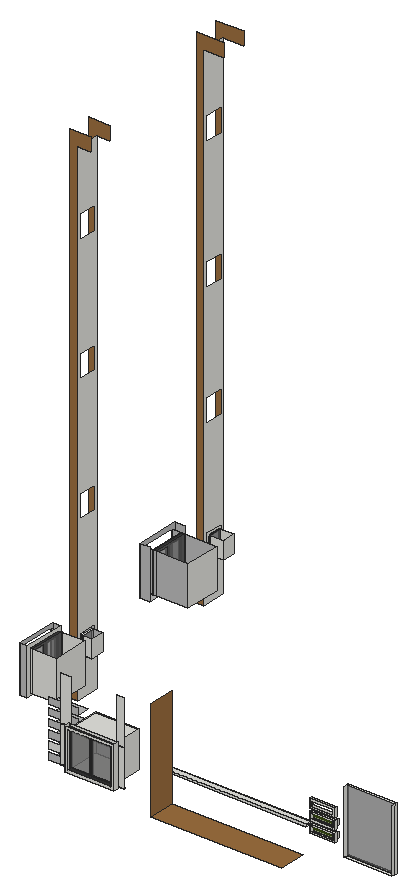
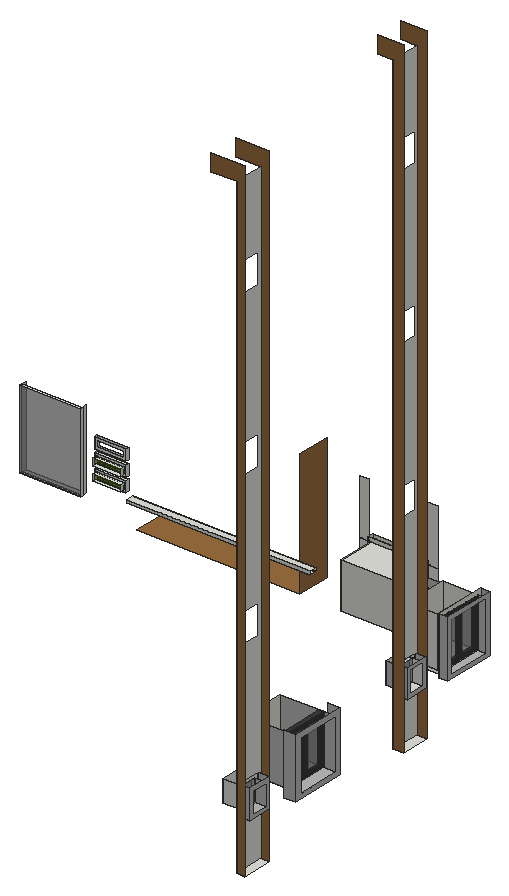
# SketchUp Ruby script. Lengths in inches.
U = 1.inch
M = Sketchup.active_model
def pt(a) = Geom::Point3d.new(a.map { |v| v * U })
def face(e, loops, mat)
  f = e.add_face(loops[0].map { |a| pt(a) })
  loops[1..].each { |l| e.add_face(l.map { |a| pt(a) }).erase! }
  f.material = f.back_material = mat if mat
  f
end
# faces: each face lists its corners as indices into pts; further lists are holes
def faces(e, pts, list, mat = nil) = list.each { |f| face(e, (f[0].is_a?(Array) ? f : [f]).map { |l| l.map { |i| pts[i] } }, mat) }
# xy, xz, yz: faces in a plane at the given z, y or x. An outline is a flat list of corners, or four numbers for a rectangle; further outlines are holes
def ring(l) = l.size == 4 ? [[l[0], l[1]], [l[2], l[1]], [l[2], l[3]], [l[0], l[3]]] : l.each_slice(2).to_a
def flat(e, list, mat, &to3) = list.each { |f| face(e, (f[0].is_a?(Array) ? f : [f]).map { |l| ring(l).map { |u, v| to3.(u, v) } }, mat) }
def xy(e, z, list, mat = nil) = flat(e, list, mat) { |x, y| [x, y, z] }
def xz(e, y, list, mat = nil) = flat(e, list, mat) { |x, z| [x, y, z] }
def yz(e, x, list, mat = nil) = flat(e, list, mat) { |y, z| [x, y, z] }
def lines(e, pts, list) = list.each { |a, b| e.add_line(pt(pts[a]), pt(pts[b])) }
# prism: a flat outline (further loops are holes) pulled along v
def prism(e, loops, v, mat = nil)
  f = face(e, loops, mat); d = Geom::Vector3d.new(v.map { |x| x * U })
  f.pushpull(f.normal.samedirection?(d) ? d.length : -d.length)
end
def box(e, o, s, mat = nil) = prism(e, [[o, [o[0] + s[0], o[1], o[2]], [o[0] + s[0], o[1] + s[1], o[2]], [o[0], o[1] + s[1], o[2]]]], [0, 0, s[2]], mat)
def at(x, y, z, deg = 0) = Geom::Transformation.translation(pt([x, y, z])) * Geom::Transformation.rotation(ORIGIN, Z_AXIS, deg.degrees)
def axes(o, x, y, z) = Geom::Transformation.new([*x, 0, *y, 0, *z, 0, *pt(o).to_a, 1])
def part(name) = M.definitions.add(name)
# library, detail: a bought-in or finely detailed component or shape, given as its bounding box
def library(name, o, s) = part(name).tap { |d| box(d.entities, o, s) }
def detail(e, o, s) = box(e.add_group.entities, o, s)
def put(e, d, t, mat = nil) = e.add_instance(d, t).tap { |i| i.material = mat if mat }
def group(e, t, mat = nil) = e.add_group.tap { |g| g.transformation = t; g.material = mat if mat }.entities
root = M.entities
M.materials.add("Generic").color = [155, 110, 63]
M.materials.add("Generic\#2").color = [186, 186, 186]
M.materials.add("[Color M07]").color = [58, 58, 58]
M.materials.add("[Translucent Glass Dark Green]").color = [62, 91, 5]
M.materials["[Translucent Glass Dark Green]"].alpha = 0.5
M.materials.add("[Translucent Glass Gray]").color = [127, 127, 127]
M.materials["[Translucent Glass Gray]"].alpha = 0.58
M.materials.add("[Translucent Glass Gray]1").color = [127, 127, 127]
M.materials["[Translucent Glass Gray]1"].alpha = 0.5
c1 = part("Group\#1")
xy(c1.entities,0,[[0,0,46.77,20.375]])
xz(c1.entities,0,[[0,0,46.77,11.0625]])
c2 = part("Group\#3")
xy(c2.entities,0,[[0,0,70.4375,6]],"[Color M07]")
xy(c2.entities,2.83,[[2.83,0,33.8,3],[36.63,0,67.61,3]],"[Color M07]")
xy(c2.entities,56.73,[[2.83,0,33.8,3],[36.63,0,67.61,3]],"[Color M07]")
xy(c2.entities,59.5625,[[0,0,70.4375,6]],"[Color M07]")
xz(c2.entities,0,[[[0,0,70.4375,59.5625],[2.83,2.83,33.8,56.73],[36.63,2.83,67.61,56.73]]],"[Color M07]")
xz(c2.entities,3,[[2.83,2.83,33.8,56.73],[36.63,2.83,67.61,56.73]],"[Translucent Glass Gray]")
xz(c2.entities,6,[[0,0,70.4375,59.5625]],"[Translucent Glass Gray]")
yz(c2.entities,0,[[0,0,6,59.5625]],"[Color M07]")
yz(c2.entities,2.83,[[0,2.83,3,56.73]],"[Color M07]")
yz(c2.entities,33.8,[[0,2.83,3,56.73]],"[Color M07]")
yz(c2.entities,36.63,[[0,2.83,3,56.73]],"[Color M07]")
yz(c2.entities,67.61,[[0,2.83,3,56.73]],"[Color M07]")
yz(c2.entities,70.4375,[[0,0,6,59.5625]],"[Color M07]")
c3 = part("Group\#7")
xy(c3.entities,0,[[0,0,36.1875,3]])
xy(c3.entities,8.75,[[0,0,36.1875,3]])
xz(c3.entities,0,[[0,0,36.1875,8.75]],"[Translucent Glass Dark Green]")
xz(c3.entities,3,[[0,0,36.1875,8.75]],"[Translucent Glass Dark Green]")
yz(c3.entities,0,[[0,0,3,8.75]])
yz(c3.entities,36.1875,[[0,0,3,8.75]])
c4 = part("Group\#4")
xy(c4.entities,0,[[0,0,6,57.4375]],"[Color M07]")
xy(c4.entities,5.48,[[0,5.48,3,25.98],[0,31.46,3,51.96]],"[Color M07]")
xy(c4.entities,59.46,[[0,5.48,3,25.98],[0,31.46,3,51.96]],"[Color M07]")
xy(c4.entities,64.9375,[[0,0,6,57.4375]],"[Color M07]")
xz(c4.entities,0,[[0,0,6,64.9375]],"[Color M07]")
xz(c4.entities,5.48,[[0,5.48,3,59.46]],"[Color M07]")
xz(c4.entities,25.98,[[0,5.48,3,59.46]],"[Color M07]")
xz(c4.entities,31.46,[[0,5.48,3,59.46]],"[Color M07]")
xz(c4.entities,51.96,[[0,5.48,3,59.46]],"[Color M07]")
xz(c4.entities,57.4375,[[0,0,6,64.9375]],"[Color M07]")
yz(c4.entities,0,[[[0,0,57.4375,64.9375],[31.46,5.48,51.96,59.46],[5.48,5.48,25.98,59.46]]],"[Color M07]")
yz(c4.entities,3,[[5.48,5.48,25.98,59.46],[31.46,5.48,51.96,59.46]],"[Translucent Glass Gray]1")
yz(c4.entities,6,[[0,0,57.4375,64.9375]],"[Translucent Glass Gray]1")
c5 = part("Group\#5")
xy(c5.entities,0,[[0,0,3,21.5625]])
xy(c5.entities,28.3125,[[0,0,3,21.5625]])
xz(c5.entities,0,[[0,0,3,28.3125]])
xz(c5.entities,21.5625,[[0,0,3,28.3125]])
yz(c5.entities,0,[[0,0,21.5625,28.3125]],"[Translucent Glass Gray]1")
yz(c5.entities,3,[[0,0,21.5625,28.3125]],"[Translucent Glass Gray]1")
xy(root,216.21,[[4.375,563.94,15.3125,603.53]])
xy(root,219.07,[[35,268.32,48.5,306.87]])
xy(root,226.375,[[315.5625,81.125,528.75,124.5]],"Generic")
xy(root,236.625,[[170.35,89.25,249.19,97.25],[172.53,97.25,173.03,98],[247.78,97.25,248.28,98.375]])
xy(root,239.9375,[[157.47,97.25,170.35,98],[249.19,97.25,259.3125,98.375]])
xy(root,240.4375,[[157.47,97.25,170.35,98],[249.19,97.25,259.3125,98.375]])
xy(root,240.83,[[174.55,89.25,244.99,97.25],[174.55,97.25,244.99,145.8125]])
xy(root,246.29,[[594.67,124.5,673.48,130.75]])
xy(root,264.83,[[[290.4375,130.75,528.75,140.05],[520.27,135.31,520.48,135.34,520.67,135.42,520.84,135.55,520.97,135.72,521.05,135.91,521.08,136.12,521.05,136.33,520.97,136.53,520.84,136.7,520.67,136.83,520.48,136.91,520.27,136.93,520.06,136.91,519.86,136.83,519.69,136.7,519.5625,136.53,519.48,136.33,519.45,136.12,519.48,135.91,519.5625,135.72,519.69,135.55,519.86,135.42,520.06,135.34],[514.2,135.31,514.41,135.34,514.61,135.42,514.78,135.55,514.91,135.72,514.99,135.91,515.02,136.12,514.99,136.33,514.91,136.53,514.78,136.7,514.61,136.83,514.41,136.91,514.2,136.93,513.99,136.91,513.8,136.83,513.63,136.7,513.5,136.53,513.42,136.33,513.39,136.12,513.42,135.91,513.5,135.72,513.63,135.55,513.8,135.42,513.99,135.34],[508.14,135.31,508.35,135.34,508.55,135.42,508.72,135.55,508.85,135.72,508.93,135.91,508.95,136.12,508.93,136.33,508.85,136.53,508.72,136.7,508.55,136.83,508.35,136.91,508.14,136.93,507.93,136.91,507.74,136.83,507.57,136.7,507.4375,136.53,507.36,136.33,507.33,136.12,507.36,135.91,507.4375,135.72,507.57,135.55,507.74,135.42,507.93,135.34],[502.27,135.31,502.48,135.34,502.67,135.42,502.84,135.55,502.97,135.72,503.05,135.91,503.08,136.12,503.05,136.33,502.97,136.53,502.84,136.7,502.67,136.83,502.48,136.91,502.27,136.93,502.06,136.91,501.86,136.83,501.69,136.7,501.5625,136.53,501.48,136.33,501.45,136.12,501.48,135.91,501.5625,135.72,501.69,135.55,501.86,135.42,502.06,135.34],[496.27,135.31,496.48,135.34,496.67,135.42,496.84,135.55,496.97,135.72,497.05,135.91,497.08,136.12,497.05,136.33,496.97,136.53,496.84,136.7,496.67,136.83,496.48,136.91,496.27,136.93,496.06,136.91,495.86,136.83,495.69,136.7,495.5625,136.53,495.48,136.33,495.45,136.12,495.48,135.91,495.5625,135.72,495.69,135.55,495.86,135.42,496.06,135.34],[490.27,135.31,490.48,135.34,490.67,135.42,490.84,135.55,490.97,135.72,491.05,135.91,491.08,136.12,491.05,136.33,490.97,136.53,490.84,136.7,490.67,136.83,490.48,136.91,490.27,136.93,490.06,136.91,489.86,136.83,489.69,136.7,489.5625,136.53,489.48,136.33,489.45,136.12,489.48,135.91,489.5625,135.72,489.69,135.55,489.86,135.42,490.06,135.34],[484.2,135.31,484.41,135.34,484.61,135.42,484.78,135.55,484.91,135.72,484.99,135.91,485.02,136.12,484.99,136.33,484.91,136.53,484.78,136.7,484.61,136.83,484.41,136.91,484.2,136.93,483.99,136.91,483.8,136.83,483.63,136.7,483.5,136.53,483.42,136.33,483.39,136.12,483.42,135.91,483.5,135.72,483.63,135.55,483.8,135.42,483.99,135.34],[478.27,135.31,478.48,135.34,478.67,135.42,478.84,135.55,478.97,135.72,479.05,135.91,479.08,136.12,479.05,136.33,478.97,136.53,478.84,136.7,478.67,136.83,478.48,136.91,478.27,136.93,478.06,136.91,477.86,136.83,477.69,136.7,477.5625,136.53,477.48,136.33,477.45,136.12,477.48,135.91,477.5625,135.72,477.69,135.55,477.86,135.42,478.06,135.34],[472.27,135.31,472.48,135.34,472.67,135.42,472.84,135.55,472.97,135.72,473.05,135.91,473.08,136.12,473.05,136.33,472.97,136.53,472.84,136.7,472.67,136.83,472.48,136.91,472.27,136.93,472.06,136.91,471.86,136.83,471.69,136.7,471.5625,136.53,471.48,136.33,471.45,136.12,471.48,135.91,471.5625,135.72,471.69,135.55,471.86,135.42,472.06,135.34],[466.27,135.31,466.48,135.34,466.67,135.42,466.84,135.55,466.97,135.72,467.05,135.91,467.08,136.12,467.05,136.33,466.97,136.53,466.84,136.7,466.67,136.83,466.48,136.91,466.27,136.93,466.06,136.91,465.86,136.83,465.69,136.7,465.5625,136.53,465.48,136.33,465.45,136.12,465.48,135.91,465.5625,135.72,465.69,135.55,465.86,135.42,466.06,135.34],[460.33,135.31,460.54,135.34,460.74,135.42,460.9,135.55,461.03,135.72,461.11,135.91,461.14,136.12,461.11,136.33,461.03,136.53,460.9,136.7,460.74,136.83,460.54,136.91,460.33,136.93,460.12,136.91,459.92,136.83,459.75,136.7,459.625,136.53,459.54,136.33,459.52,136.12,459.54,135.91,459.625,135.72,459.75,135.55,459.92,135.42,460.12,135.34],[454.33,135.31,454.54,135.34,454.74,135.42,454.9,135.55,455.03,135.72,455.11,135.91,455.14,136.12,455.11,136.33,455.03,136.53,454.9,136.7,454.74,136.83,454.54,136.91,454.33,136.93,454.12,136.91,453.92,136.83,453.75,136.7,453.625,136.53,453.54,136.33,453.52,136.12,453.54,135.91,453.625,135.72,453.75,135.55,453.92,135.42,454.12,135.34],[448.33,135.31,448.54,135.34,448.74,135.42,448.9,135.55,449.03,135.72,449.11,135.91,449.14,136.12,449.11,136.33,449.03,136.53,448.9,136.7,448.74,136.83,448.54,136.91,448.33,136.93,448.12,136.91,447.92,136.83,447.75,136.7,447.625,136.53,447.54,136.33,447.52,136.12,447.54,135.91,447.625,135.72,447.75,135.55,447.92,135.42,448.12,135.34],[442.33,135.31,442.54,135.34,442.74,135.42,442.9,135.55,443.03,135.72,443.11,135.91,443.14,136.12,443.11,136.33,443.03,136.53,442.9,136.7,442.74,136.83,442.54,136.91,442.33,136.93,442.12,136.91,441.92,136.83,441.75,136.7,441.625,136.53,441.54,136.33,441.52,136.12,441.54,135.91,441.625,135.72,441.75,135.55,441.92,135.42,442.12,135.34],[436.33,135.31,436.54,135.34,436.74,135.42,436.9,135.55,437.03,135.72,437.11,135.91,437.14,136.12,437.11,136.33,437.03,136.53,436.9,136.7,436.74,136.83,436.54,136.91,436.33,136.93,436.12,136.91,435.92,136.83,435.75,136.7,435.625,136.53,435.54,136.33,435.52,136.12,435.54,135.91,435.625,135.72,435.75,135.55,435.92,135.42,436.12,135.34],[430.33,135.31,430.54,135.34,430.74,135.42,430.9,135.55,431.03,135.72,431.11,135.91,431.14,136.12,431.11,136.33,431.03,136.53,430.9,136.7,430.74,136.83,430.54,136.91,430.33,136.93,430.12,136.91,429.92,136.83,429.75,136.7,429.625,136.53,429.54,136.33,429.52,136.12,429.54,135.91,429.625,135.72,429.75,135.55,429.92,135.42,430.12,135.34],[424.33,135.31,424.54,135.34,424.74,135.42,424.9,135.55,425.03,135.72,425.11,135.91,425.14,136.12,425.11,136.33,425.03,136.53,424.9,136.7,424.74,136.83,424.54,136.91,424.33,136.93,424.12,136.91,423.92,136.83,423.75,136.7,423.625,136.53,423.54,136.33,423.52,136.12,423.54,135.91,423.625,135.72,423.75,135.55,423.92,135.42,424.12,135.34],[418.33,135.31,418.54,135.34,418.74,135.42,418.9,135.55,419.03,135.72,419.11,135.91,419.14,136.12,419.11,136.33,419.03,136.53,418.9,136.7,418.74,136.83,418.54,136.91,418.33,136.93,418.12,136.91,417.92,136.83,417.75,136.7,417.625,136.53,417.54,136.33,417.52,136.12,417.54,135.91,417.625,135.72,417.75,135.55,417.92,135.42,418.12,135.34],[412.33,135.31,412.54,135.34,412.74,135.42,412.9,135.55,413.03,135.72,413.11,135.91,413.14,136.12,413.11,136.33,413.03,136.53,412.9,136.7,412.74,136.83,412.54,136.91,412.33,136.93,412.12,136.91,411.92,136.83,411.75,136.7,411.625,136.53,411.54,136.33,411.52,136.12,411.54,135.91,411.625,135.72,411.75,135.55,411.92,135.42,412.12,135.34],[406.33,135.31,406.54,135.34,406.74,135.42,406.9,135.55,407.03,135.72,407.11,135.91,407.14,136.12,407.11,136.33,407.03,136.53,406.9,136.7,406.74,136.83,406.54,136.91,406.33,136.93,406.12,136.91,405.92,136.83,405.75,136.7,405.625,136.53,405.54,136.33,405.52,136.12,405.54,135.91,405.625,135.72,405.75,135.55,405.92,135.42,406.12,135.34],[400.33,135.31,400.54,135.34,400.74,135.42,400.9,135.55,401.03,135.72,401.11,135.91,401.14,136.12,401.11,136.33,401.03,136.53,400.9,136.7,400.74,136.83,400.54,136.91,400.33,136.93,400.12,136.91,399.92,136.83,399.75,136.7,399.625,136.53,399.54,136.33,399.52,136.12,399.54,135.91,399.625,135.72,399.75,135.55,399.92,135.42,400.12,135.34],[394.2,135.31,394.41,135.34,394.61,135.42,394.78,135.55,394.91,135.72,394.99,135.91,395.02,136.12,394.99,136.33,394.91,136.53,394.78,136.7,394.61,136.83,394.41,136.91,394.2,136.93,393.99,136.91,393.8,136.83,393.63,136.7,393.5,136.53,393.42,136.33,393.39,136.12,393.42,135.91,393.5,135.72,393.63,135.55,393.8,135.42,393.99,135.34],[388.08,135.31,388.29,135.34,388.49,135.42,388.65,135.55,388.78,135.72,388.86,135.91,388.89,136.12,388.86,136.33,388.78,136.53,388.65,136.7,388.49,136.83,388.29,136.91,388.08,136.93,387.87,136.91,387.67,136.83,387.5,136.7,387.375,136.53,387.29,136.33,387.27,136.12,387.29,135.91,387.375,135.72,387.5,135.55,387.67,135.42,387.87,135.34],[382.27,135.31,382.48,135.34,382.67,135.42,382.84,135.55,382.97,135.72,383.05,135.91,383.08,136.12,383.05,136.33,382.97,136.53,382.84,136.7,382.67,136.83,382.48,136.91,382.27,136.93,382.06,136.91,381.86,136.83,381.69,136.7,381.5625,136.53,381.48,136.33,381.45,136.12,381.48,135.91,381.5625,135.72,381.69,135.55,381.86,135.42,382.06,135.34],[376.27,135.31,376.48,135.34,376.67,135.42,376.84,135.55,376.97,135.72,377.05,135.91,377.08,136.12,377.05,136.33,376.97,136.53,376.84,136.7,376.67,136.83,376.48,136.91,376.27,136.93,376.06,136.91,375.86,136.83,375.69,136.7,375.5625,136.53,375.48,136.33,375.45,136.12,375.48,135.91,375.5625,135.72,375.69,135.55,375.86,135.42,376.06,135.34],[370.2,135.31,370.41,135.34,370.61,135.42,370.78,135.55,370.91,135.72,370.99,135.91,371.02,136.12,370.99,136.33,370.91,136.53,370.78,136.7,370.61,136.83,370.41,136.91,370.2,136.93,369.99,136.91,369.8,136.83,369.63,136.7,369.5,136.53,369.42,136.33,369.39,136.12,369.42,135.91,369.5,135.72,369.63,135.55,369.8,135.42,369.99,135.34],[364.27,135.31,364.48,135.34,364.67,135.42,364.84,135.55,364.97,135.72,365.05,135.91,365.08,136.12,365.05,136.33,364.97,136.53,364.84,136.7,364.67,136.83,364.48,136.91,364.27,136.93,364.06,136.91,363.86,136.83,363.69,136.7,363.5625,136.53,363.48,136.33,363.45,136.12,363.48,135.91,363.5625,135.72,363.69,135.55,363.86,135.42,364.06,135.34],[358.27,135.31,358.48,135.34,358.67,135.42,358.84,135.55,358.97,135.72,359.05,135.91,359.08,136.12,359.05,136.33,358.97,136.53,358.84,136.7,358.67,136.83,358.48,136.91,358.27,136.93,358.06,136.91,357.86,136.83,357.69,136.7,357.5625,136.53,357.48,136.33,357.45,136.12,357.48,135.91,357.5625,135.72,357.69,135.55,357.86,135.42,358.06,135.34],[352.27,135.31,352.48,135.34,352.67,135.42,352.84,135.55,352.97,135.72,353.05,135.91,353.08,136.12,353.05,136.33,352.97,136.53,352.84,136.7,352.67,136.83,352.48,136.91,352.27,136.93,352.06,136.91,351.86,136.83,351.69,136.7,351.5625,136.53,351.48,136.33,351.45,136.12,351.48,135.91,351.5625,135.72,351.69,135.55,351.86,135.42,352.06,135.34],[346.27,135.31,346.48,135.34,346.67,135.42,346.84,135.55,346.97,135.72,347.05,135.91,347.08,136.12,347.05,136.33,346.97,136.53,346.84,136.7,346.67,136.83,346.48,136.91,346.27,136.93,346.06,136.91,345.86,136.83,345.69,136.7,345.5625,136.53,345.48,136.33,345.45,136.12,345.48,135.91,345.5625,135.72,345.69,135.55,345.86,135.42,346.06,135.34],[340.27,135.31,340.48,135.34,340.67,135.42,340.84,135.55,340.97,135.72,341.05,135.91,341.08,136.12,341.05,136.33,340.97,136.53,340.84,136.7,340.67,136.83,340.48,136.91,340.27,136.93,340.06,136.91,339.86,136.83,339.69,136.7,339.5625,136.53,339.48,136.33,339.45,136.12,339.48,135.91,339.5625,135.72,339.69,135.55,339.86,135.42,340.06,135.34],[334.27,135.31,334.48,135.34,334.67,135.42,334.84,135.55,334.97,135.72,335.05,135.91,335.08,136.12,335.05,136.33,334.97,136.53,334.84,136.7,334.67,136.83,334.48,136.91,334.27,136.93,334.06,136.91,333.86,136.83,333.69,136.7,333.5625,136.53,333.48,136.33,333.45,136.12,333.48,135.91,333.5625,135.72,333.69,135.55,333.86,135.42,334.06,135.34],[328.27,135.31,328.48,135.34,328.67,135.42,328.84,135.55,328.97,135.72,329.05,135.91,329.08,136.12,329.05,136.33,328.97,136.53,328.84,136.7,328.67,136.83,328.48,136.91,328.27,136.93,328.06,136.91,327.86,136.83,327.69,136.7,327.5625,136.53,327.48,136.33,327.45,136.12,327.48,135.91,327.5625,135.72,327.69,135.55,327.86,135.42,328.06,135.34],[322.27,135.31,322.48,135.34,322.67,135.42,322.84,135.55,322.97,135.72,323.05,135.91,323.08,136.12,323.05,136.33,322.97,136.53,322.84,136.7,322.67,136.83,322.48,136.91,322.27,136.93,322.06,136.91,321.86,136.83,321.69,136.7,321.5625,136.53,321.48,136.33,321.45,136.12,321.48,135.91,321.5625,135.72,321.69,135.55,321.86,135.42,322.06,135.34],[316.27,135.31,316.48,135.34,316.67,135.42,316.84,135.55,316.97,135.72,317.05,135.91,317.08,136.12,317.05,136.33,316.97,136.53,316.84,136.7,316.67,136.83,316.48,136.91,316.27,136.93,316.06,136.91,315.86,136.83,315.69,136.7,315.5625,136.53,315.48,136.33,315.45,136.12,315.48,135.91,315.5625,135.72,315.69,135.55,315.86,135.42,316.06,135.34],[310.27,135.31,310.48,135.34,310.67,135.42,310.84,135.55,310.97,135.72,311.05,135.91,311.08,136.12,311.05,136.33,310.97,136.53,310.84,136.7,310.67,136.83,310.48,136.91,310.27,136.93,310.06,136.91,309.86,136.83,309.69,136.7,309.5625,136.53,309.48,136.33,309.45,136.12,309.48,135.91,309.5625,135.72,309.69,135.55,309.86,135.42,310.06,135.34],[303.89,135.31,304.1,135.34,304.3,135.42,304.47,135.55,304.6,135.72,304.68,135.91,304.7,136.12,304.68,136.33,304.6,136.53,304.47,136.7,304.3,136.83,304.1,136.91,303.89,136.93,303.68,136.91,303.49,136.83,303.32,136.7,303.1875,136.53,303.11,136.33,303.08,136.12,303.11,135.91,303.1875,135.72,303.32,135.55,303.49,135.42,303.68,135.34]]])
xy(root,265.07,[[542.55,120,583.96,124.5]])
xy(root,267.68,[[545.16,120,581.35,124.5],[545.16,124.5,581.35,130.75]])
xy(root,269.02,[[290.4375,130.75,528.75,140.05]])
xy(root,269.52,[[37,164.2,48.5,231.93]],"Generic\#2")
xy(root,270.33,[[0,454.08,15.3125,525.8]],"Generic\#2")
xy(root,274.66,[[48.5,169.34,93.0625,226.78]])
xy(root,274.66,[[37,169.34,48.5,226.78]],"Generic\#2")
xy(root,276.43,[[545.16,120,581.35,124.5],[545.16,124.5,581.35,130.75]])
xy(root,277.48,[[0,461.22,72.5625,518.66]],"Generic\#2")
xy(root,279.04,[[542.55,120,583.96,124.5]])
xy(root,279.42,[[34.5,270.92,48.5,300.91]],"Generic\#2")
xy(root,281.36,[[0,569.42,15.3125,600.66]],"Generic\#2")
xy(root,283.57,[[542.55,120,583.96,124.5]])
xy(root,283.64,[[34.5,275.13,65.625,296.69]])
xy(root,286.18,[[545.16,120,581.35,124.5],[545.16,124.5,581.35,130.75]])
xy(root,286.2,[[15.3125,574.26,39.625,595.82]])
xy(root,286.2,[[0,574.26,15.3125,595.82]],"Generic\#2")
xy(root,294.93,[[545.16,120,581.35,124.5],[545.16,124.5,581.35,130.75]])
xy(root,297.54,[[542.55,120,583.96,124.5]])
xy(root,300.39,[[174.55,89.25,244.99,97.25],[174.55,97.25,244.99,145.8125]])
xy(root,302.07,[[542.55,120,583.96,124.5]])
xz(root,89.25,[[[170.35,236.625,249.19,304.59],[174.55,240.83,244.99,300.39]]])
xz(root,97.25,[[170.35,236.625,172.53,240.4375],[172.53,236.625,248.28,240.4375],[248.28,236.625,249.19,240.4375],[157.47,240.4375,170.35,299.625],[170.35,240.4375,172.53,300.125],
  [172.53,240.4375,172.53,300.125,174.55,300.125,174.55,240.83,244.99,240.83,244.99,300.125,248.28,300.125,248.28,240.4375],[248.28,240.4375,249.19,300.125],[249.19,240.4375,259.3125,299.625],[157.47,299.625,170.35,300.125],[249.19,299.625,259.3125,300.125],
  [157.47,300.125,170.35,300.125,170.35,304.59,172.53,304.59,172.53,372.9375,157.47,372.9375],[170.35,300.125,172.53,304.59],[172.53,300.125,172.53,304.59,248.28,304.59,248.28,300.125,244.99,300.125,244.99,300.39,174.55,300.39,174.55,300.125],[248.28,300.125,249.19,304.59],[249.19,300.125,259.3125,300.125,259.3125,372.9375,248.28,372.9375,248.28,304.59,249.19,304.59]])
xz(root,98,[[157.47,239.9375,170.35,240.4375]])
xz(root,98.375,[[249.19,239.9375,259.3125,240.4375]])
xz(root,120,[[[542.55,265.07,583.96,279.04],[545.16,267.68,581.35,276.43]],[[542.55,283.57,583.96,297.54],[545.16,286.18,581.35,294.93]],[[542.55,302.07,583.96,316.04],[545.16,304.68,581.35,313.43]]])
xz(root,124.5,[[[542.55,265.07,583.96,279.04],[545.16,267.68,581.35,276.43]],[[542.55,283.57,583.96,297.54],[545.16,286.18,581.35,294.93]],[[542.55,302.07,583.96,316.04],[545.16,304.68,581.35,313.43]]])
xz(root,130.75,[[290.4375,264.83,528.75,269.02]])
xz(root,140.05,[[290.4375,264.83,528.75,269.02]])
xz(root,145.8125,[[174.55,240.83,244.99,300.39]])
xz(root,164.2,[[37,269.52,48.5,344.75]],"Generic\#2")
xz(root,169.34,[[48.5,274.66,93.0625,339.6]])
xz(root,169.34,[[37,274.66,48.5,339.6]],"Generic\#2")
xz(root,226.78,[[48.5,274.66,93.0625,339.6]])
xz(root,226.78,[[37,274.66,48.5,339.6]],"Generic\#2")
xz(root,231.93,[[37,269.52,48.5,344.75]],"Generic\#2")
xz(root,268.32,[[35,219.07,35,1046.8125,69,1046.8125,69,1024.6875,48.5,1024.6875,48.5,219.07]],"Generic")
xz(root,270.92,[[34.5,279.42,48.5,316.16]],"Generic\#2")
xz(root,275.13,[[34.5,283.64,65.625,311.95]])
xz(root,296.69,[[34.5,283.64,65.625,311.95]],"Generic\#2")
xz(root,300.91,[[34.5,279.42,48.5,316.16]],"Generic\#2")
xz(root,306.87,[[35,219.07,48.5,219.07,48.5,1024.6875,69,1024.6875,69,1046.8125,35,1046.8125]],"Generic")
xz(root,454.08,[[0,270.33,15.3125,349.56]],"Generic\#2")
xz(root,461.22,[[0,277.48,72.5625,342.41]],"Generic\#2")
xz(root,518.66,[[0,277.48,72.5625,342.41]],"Generic\#2")
xz(root,525.8,[[0,270.33,15.3125,349.56]],"Generic\#2")
xz(root,563.94,[[4.375,216.21,4.375,1046.8125,48.5,1046.8125,48.5,1024.6875,15.3125,1024.6875,15.3125,216.21]],"Generic")
xz(root,569.42,[[0,281.36,15.3125,319.35]],"Generic\#2")
xz(root,574.26,[[15.3125,286.2,39.625,314.51]])
xz(root,574.26,[[0,286.2,15.3125,314.51]],"Generic\#2")
xz(root,595.82,[[15.3125,286.2,39.625,314.51]])
xz(root,595.82,[[0,286.2,15.3125,314.51]],"Generic\#2")
xz(root,600.66,[[0,281.36,15.3125,319.35]],"Generic\#2")
xz(root,603.53,[[4.375,216.21,15.3125,216.21,15.3125,1024.6875,48.5,1024.6875,48.5,1046.8125,4.375,1046.8125]],"Generic")
yz(root,0,[[[454.08,270.33,525.8,349.56],[461.22,277.48,518.66,342.41]],[[569.42,281.36,600.66,319.35],[574.26,286.2,595.82,314.51]]],"Generic\#2")
yz(root,15.3125,[[[563.94,216.21,603.53,1024.6875],[569.11,888.61,600.97,927.22],[569.11,675.92,600.66,714.22],[569.42,478.92,600.66,516.91],[569.42,281.36,600.66,319.35]],[[569.42,281.36,600.66,319.35],[574.26,286.2,595.82,314.51]]])
yz(root,34.5,[[[270.92,279.42,300.91,316.16],[275.13,283.64,296.69,311.95]]],"Generic\#2")
yz(root,37,[[[164.2,269.52,231.93,344.75],[169.34,274.66,226.78,339.6]]],"Generic\#2")
yz(root,39.625,[[574.26,286.2,595.82,314.51]])
yz(root,48.5,[[[268.32,219.07,306.87,1024.6875],[270.92,889.11,300.91,926.29],[270.92,686.17,300.91,722.91],[270.92,482.8,300.91,519.54],[270.92,279.42,300.91,316.16]],[[164.2,269.52,231.93,344.75],[169.34,274.66,226.78,339.6]]])
yz(root,65.625,[[275.13,283.64,296.69,311.95]])
yz(root,72.5625,[[461.22,277.48,518.66,342.41]])
yz(root,93.0625,[[169.34,274.66,226.78,339.6]])
yz(root,170.35,[[89.25,236.625,97.25,304.59],[97.25,239.9375,98,240.4375]])
yz(root,174.55,[[89.25,240.83,97.25,300.39],[97.25,240.83,145.8125,300.39]])
yz(root,244.99,[[89.25,240.83,97.25,300.39],[97.25,240.83,145.8125,300.39]])
yz(root,249.19,[[89.25,236.625,97.25,304.59],[97.25,239.9375,98.375,240.4375]])
yz(root,315.5625,[[81.125,226.375,124.5,390.1875]],"Generic")
yz(root,542.55,[[120,265.07,124.5,279.04],[120,283.57,124.5,297.54],[120,302.07,124.5,316.04]])
yz(root,545.16,[[120,267.68,124.5,276.43],[124.5,267.68,130.75,276.43],[120,286.18,124.5,294.93],[124.5,286.18,130.75,294.93]])
yz(root,581.35,[[120,267.68,124.5,276.43],[124.5,267.68,130.75,276.43],[120,286.18,124.5,294.93],[124.5,286.18,130.75,294.93]])
yz(root,583.96,[[120,265.07,124.5,279.04],[120,283.57,124.5,297.54],[120,302.07,124.5,316.04]])
yz(root,594.67,[[124.5,246.29,130.75,349.35]])
yz(root,673.48,[[124.5,246.29,130.75,349.35]])
p = [[528.75,134.84,266.52],[290.4375,134.84,266.52],[244.99,97.25,300.125],[174.55,97.25,300.125]]
lines(root,p,[[0,1],[2,3]])
put(root,c1,at(110.7,130.3125,215.875),"Generic\#2")
put(root,c1,at(110.7,130.3125,232.0625))
put(root,c2,at(174.55,91.75,240.83))
g1 = group(root,at(594.67,130.75,246.29))
xy(g1,0,[[0,0,78.8125,3]])
xy(g1,103.0625,[[0,0,78.8125,3]])
xz(g1,0,[[0,0,78.8125,103.0625]],"[Translucent Glass Gray]1")
xz(g1,3,[[0,0,78.8125,103.0625]],"[Translucent Glass Gray]1")
yz(g1,0,[[0,0,3,103.0625]])
yz(g1,78.8125,[[0,0,3,103.0625]])
put(root,c1,at(110.7,130.3125,248.25),"Generic\#2")
put(root,c1,at(110.7,130.3125,264.4375),"Generic\#2")
put(root,c3,at(545.16,124.5,267.68))
put(root,c4,at(48.5,169.34,274.66))
put(root,c4,at(15.3125,461.22,277.48))
put(root,c1,at(110.7,130.3125,280.625),"Generic\#2")
put(root,c5,at(48.5,275.13,283.64))
put(root,c3,at(545.16,124.5,286.18))
put(root,c5,at(15.3125,574.26,286.2))
put(root,c1,at(110.7,130.3125,296.8125),"Generic\#2")
